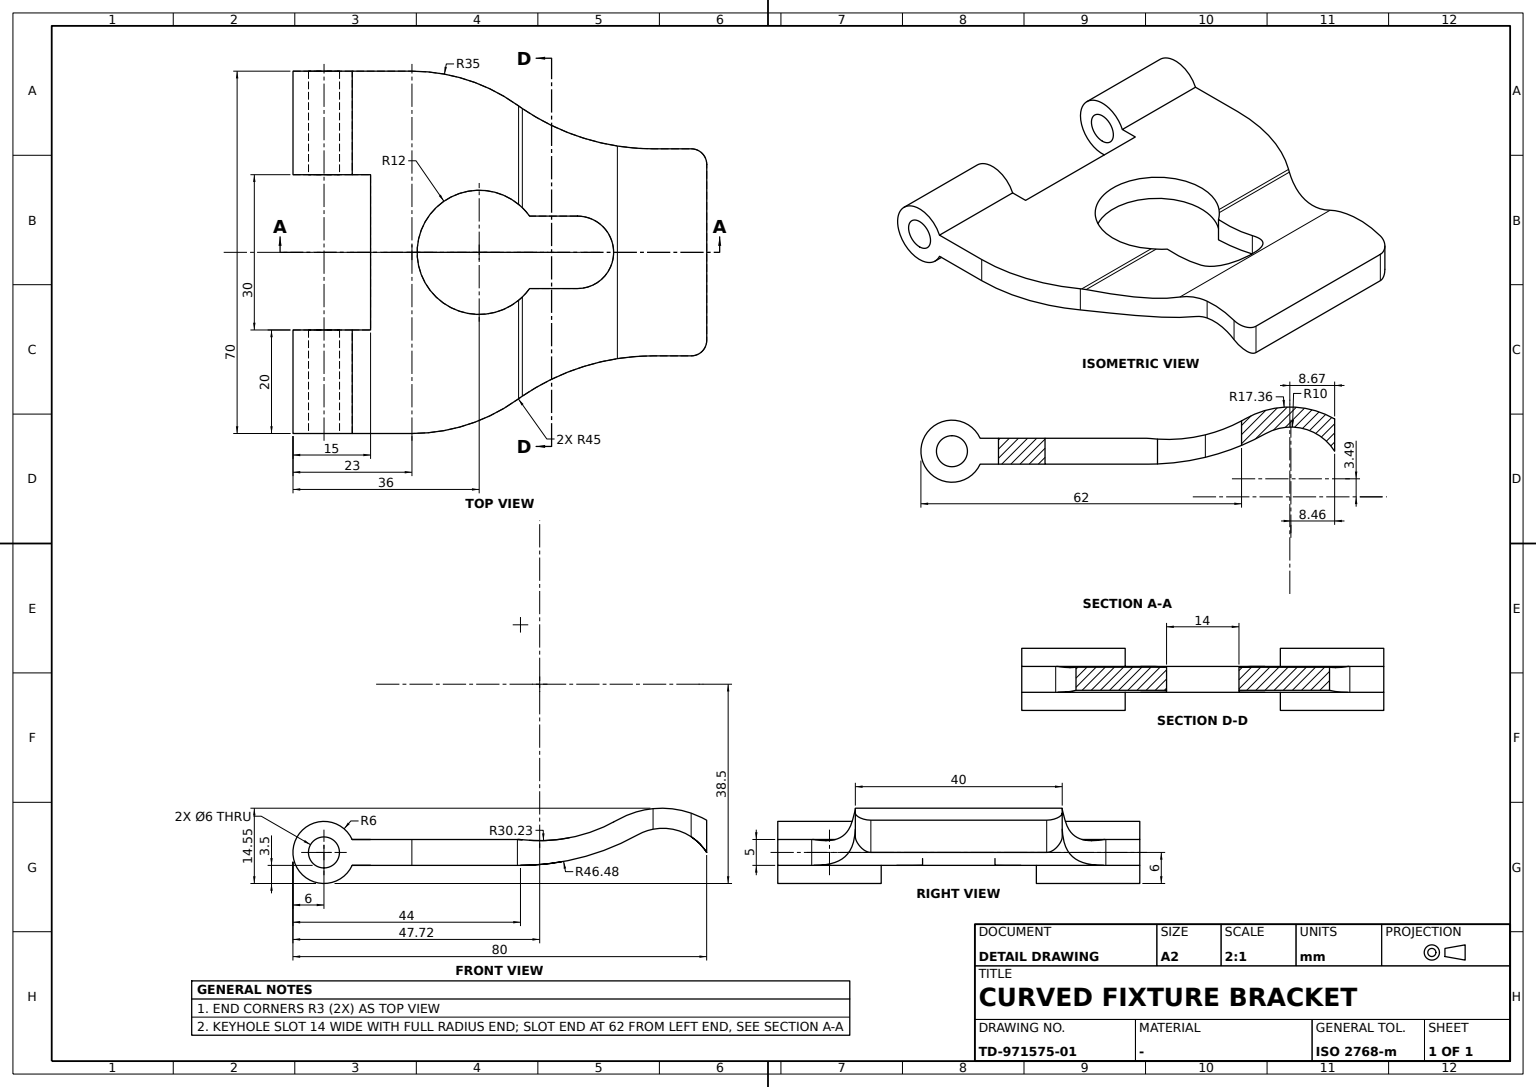
ISO-10303-21;
HEADER;
FILE_DESCRIPTION((''),'2;1');
FILE_NAME('','',(''),(''),'','','');
FILE_SCHEMA(('AUTOMOTIVE_DESIGN'));
ENDSEC;
DATA;
#1=APPLICATION_CONTEXT('');
#2=PRODUCT_CONTEXT('',#1,'mechanical');
#3=PRODUCT('','','',(#2));
#4=PRODUCT_DEFINITION_FORMATION('','',#3);
#5=PRODUCT_DEFINITION_CONTEXT('',#1,'design');
#6=PRODUCT_DEFINITION('','',#4,#5);
#7=PRODUCT_DEFINITION_SHAPE('','',#6);
#8=(LENGTH_UNIT()NAMED_UNIT(*)SI_UNIT(.MILLI.,.METRE.));
#9=(NAMED_UNIT(*)PLANE_ANGLE_UNIT()SI_UNIT($,.RADIAN.));
#10=(NAMED_UNIT(*)SI_UNIT($,.STERADIAN.)SOLID_ANGLE_UNIT());
#11=UNCERTAINTY_MEASURE_WITH_UNIT(LENGTH_MEASURE(0.005),#8,'distance_accuracy_value','');
#12=(GEOMETRIC_REPRESENTATION_CONTEXT(3)GLOBAL_UNCERTAINTY_ASSIGNED_CONTEXT((#11))GLOBAL_UNIT_ASSIGNED_CONTEXT((#8,#9,#10))REPRESENTATION_CONTEXT('',''));
#13=CARTESIAN_POINT('',(-28.4375,-36.596358,-2.5));
#14=VERTEX_POINT('',#13);
#15=CARTESIAN_POINT('',(-35.,-57.,-2.5));
#16=VERTEX_POINT('',#15);
#17=CARTESIAN_POINT('',(0.,-57.,-2.5));
#18=DIRECTION('',(0.,0.,1.));
#19=DIRECTION('',(1.,0.,0.));
#20=AXIS2_PLACEMENT_3D('',#17,#18,#19);
#21=CIRCLE('',#20,35.);
#22=EDGE_CURVE('',#14,#16,#21,.T.);
#23=ORIENTED_EDGE('',*,*,#22,.T.);
#24=CARTESIAN_POINT('',(-35.,-57.,2.5));
#25=VERTEX_POINT('',#24);
#26=CARTESIAN_POINT('',(-35.,-57.,0.));
#27=VECTOR('',#18,1000.);
#28=LINE('',#26,#27);
#29=EDGE_CURVE('',#16,#25,#28,.T.);
#30=ORIENTED_EDGE('',*,*,#29,.T.);
#31=CARTESIAN_POINT('',(-28.4375,-36.596358,2.5));
#32=VERTEX_POINT('',#31);
#33=CARTESIAN_POINT('',(0.,-57.,2.5));
#34=DIRECTION('',(0.,0.,-1.));
#35=DIRECTION('',(-1.,0.,0.));
#36=AXIS2_PLACEMENT_3D('',#33,#34,#35);
#37=CIRCLE('',#36,35.);
#38=EDGE_CURVE('',#25,#32,#37,.T.);
#39=ORIENTED_EDGE('',*,*,#38,.T.);
#40=CARTESIAN_POINT('',(-28.4375,-36.596358,0.));
#41=LINE('',#40,#27);
#42=EDGE_CURVE('',#14,#32,#41,.T.);
#43=ORIENTED_EDGE('',*,*,#42,.F.);
#44=EDGE_LOOP('',(#23,#30,#39,#43));
#45=FACE_BOUND('',#44,.T.);
#46=CARTESIAN_POINT('',(0.,-57.,0.));
#47=AXIS2_PLACEMENT_3D('',#46,#18,#19);
#48=CYLINDRICAL_SURFACE('',#47,35.);
#49=ADVANCED_FACE('',(#45),#48,.T.);
#50=CARTESIAN_POINT('',(-28.016901,-36.,-2.5));
#51=VERTEX_POINT('',#50);
#52=CARTESIAN_POINT('',(-65.,-10.363105,-2.5));
#53=AXIS2_PLACEMENT_3D('',#52,#18,#19);
#54=CIRCLE('',#53,45.);
#55=EDGE_CURVE('',#14,#51,#54,.T.);
#56=ORIENTED_EDGE('',*,*,#55,.F.);
#57=ORIENTED_EDGE('',*,*,#42,.T.);
#58=CARTESIAN_POINT('',(-28.283906,-36.380954,2.5));
#59=VERTEX_POINT('',#58);
#60=CARTESIAN_POINT('',(-65.,-10.363105,2.5));
#61=AXIS2_PLACEMENT_3D('',#60,#34,#35);
#62=CIRCLE('',#61,45.);
#63=EDGE_CURVE('',#59,#32,#62,.T.);
#64=ORIENTED_EDGE('',*,*,#63,.F.);
#65=CARTESIAN_POINT('',(-27.781293,-35.656737,2.459472));
#66=VERTEX_POINT('',#65);
#67=CARTESIAN_POINT('',(-27.946111,-35.899262,2.486701));
#68=CARTESIAN_POINT('',(-28.113645,-36.140683,2.5));
#69=B_SPLINE_CURVE_WITH_KNOTS('',3,(#65,#67,#68,#58),.UNSPECIFIED.,.F.,.F.,(4,4),(0.,0.00088247),.UNSPECIFIED.);
#70=EDGE_CURVE('',#66,#59,#69,.T.);
#71=ORIENTED_EDGE('',*,*,#70,.F.);
#72=CARTESIAN_POINT('',(-20.535037,-17.281708,6.256147));
#73=VERTEX_POINT('',#72);
#74=CARTESIAN_POINT('',(-20.766814,-18.771309,5.404617));
#75=CARTESIAN_POINT('',(-21.390954,-21.813993,3.995167));
#76=CARTESIAN_POINT('',(-23.441277,-28.200086,2.238521));
#77=CARTESIAN_POINT('',(-25.845824,-32.808762,2.139722));
#78=B_SPLINE_CURVE_WITH_KNOTS('',3,(#72,#74,#75,#76,#77,#65),.UNSPECIFIED.,.F.,.F.,(4,1,1,4),(0.,0.005116503,0.010233007,0.020466013),.UNSPECIFIED.);
#79=EDGE_CURVE('',#73,#66,#78,.T.);
#80=ORIENTED_EDGE('',*,*,#79,.F.);
#81=CARTESIAN_POINT('',(-20.,-10.363105,8.461947));
#82=VERTEX_POINT('',#81);
#83=CARTESIAN_POINT('',(-20.205135,-15.161472,7.46818));
#84=CARTESIAN_POINT('',(-20.,-12.817021,8.220804));
#85=B_SPLINE_CURVE_WITH_KNOTS('',3,(#72,#83,#84,#81),.UNSPECIFIED.,.F.,.F.,(4,4),(0.,0.007291634),.UNSPECIFIED.);
#86=EDGE_CURVE('',#73,#82,#85,.T.);
#87=ORIENTED_EDGE('',*,*,#86,.T.);
#88=CARTESIAN_POINT('',(-20.,-10.363105,4.486691));
#89=VERTEX_POINT('',#88);
#90=CARTESIAN_POINT('',(-20.,-10.363105,0.));
#91=LINE('',#90,#27);
#92=EDGE_CURVE('',#89,#82,#91,.T.);
#93=ORIENTED_EDGE('',*,*,#92,.F.);
#94=CARTESIAN_POINT('',(-20.098366,-13.336862,3.399904));
#95=VERTEX_POINT('',#94);
#96=CARTESIAN_POINT('',(-20.036616,-12.404486,3.920648));
#97=CARTESIAN_POINT('',(-20.,-11.413451,4.283158));
#98=B_SPLINE_CURVE_WITH_KNOTS('',3,(#94,#96,#97,#88),.UNSPECIFIED.,.F.,.F.,(4,4),(0.,0.003167651),.UNSPECIFIED.);
#99=EDGE_CURVE('',#95,#89,#98,.T.);
#100=ORIENTED_EDGE('',*,*,#99,.F.);
#101=CARTESIAN_POINT('',(-20.221084,-15.189824,2.365002));
#102=CARTESIAN_POINT('',(-20.6967,-18.956801,0.58839));
#103=CARTESIAN_POINT('',(-22.765086,-26.825025,-1.902632));
#104=CARTESIAN_POINT('',(-25.595054,-32.506308,-2.5));
#105=B_SPLINE_CURVE_WITH_KNOTS('',3,(#94,#101,#102,#103,#104,#50),.UNSPECIFIED.,.F.,.F.,(4,1,1,4),(0.,0.006286934,0.012573868,0.025147736),.UNSPECIFIED.);
#106=EDGE_CURVE('',#95,#51,#105,.T.);
#107=ORIENTED_EDGE('',*,*,#106,.T.);
#108=EDGE_LOOP('',(#56,#57,#64,#71,#80,#87,#93,#100,#107));
#109=FACE_BOUND('',#108,.T.);
#110=CARTESIAN_POINT('',(-65.,-10.363105,0.));
#111=AXIS2_PLACEMENT_3D('',#110,#18,#19);
#112=CYLINDRICAL_SURFACE('',#111,45.);
#113=ADVANCED_FACE('',(#109),#112,.F.);
#114=CARTESIAN_POINT('',(35.,-74.,-3.));
#115=VERTEX_POINT('',#114);
#116=CARTESIAN_POINT('',(35.,-74.,0.));
#117=AXIS2_PLACEMENT_3D('',#116,#19,#34);
#118=CIRCLE('',#117,3.);
#119=EDGE_CURVE('',#115,#115,#118,.T.);
#120=ORIENTED_EDGE('',*,*,#119,.F.);
#121=EDGE_LOOP('',(#120));
#122=FACE_BOUND('',#121,.T.);
#123=CARTESIAN_POINT('',(35.,-68.545644,2.5));
#124=VERTEX_POINT('',#123);
#125=CARTESIAN_POINT('',(35.,-57.,2.5));
#126=VERTEX_POINT('',#125);
#127=CARTESIAN_POINT('',(35.,-80.,2.5));
#128=DIRECTION('',(0.,1.,0.));
#129=VECTOR('',#128,1000.);
#130=LINE('',#127,#129);
#131=EDGE_CURVE('',#124,#126,#130,.T.);
#132=ORIENTED_EDGE('',*,*,#131,.F.);
#133=CARTESIAN_POINT('',(35.,-68.545644,-2.5));
#134=VERTEX_POINT('',#133);
#135=CIRCLE('',#117,6.);
#136=EDGE_CURVE('',#124,#134,#135,.T.);
#137=ORIENTED_EDGE('',*,*,#136,.T.);
#138=CARTESIAN_POINT('',(35.,-57.,-2.5));
#139=VERTEX_POINT('',#138);
#140=CARTESIAN_POINT('',(35.,-36.,-2.5));
#141=LINE('',#140,#129);
#142=EDGE_CURVE('',#134,#139,#141,.T.);
#143=ORIENTED_EDGE('',*,*,#142,.T.);
#144=CARTESIAN_POINT('',(35.,-57.,0.));
#145=LINE('',#144,#27);
#146=EDGE_CURVE('',#139,#126,#145,.T.);
#147=ORIENTED_EDGE('',*,*,#146,.T.);
#148=EDGE_LOOP('',(#132,#137,#143,#147));
#149=FACE_BOUND('',#148,.T.);
#150=CARTESIAN_POINT('',(35.,-80.,0.));
#151=AXIS2_PLACEMENT_3D('',#150,#19,#128);
#152=PLANE('',#151);
#153=ADVANCED_FACE('',(#122,#149),#152,.T.);
#154=CARTESIAN_POINT('',(7.,-34.253206,-2.467163));
#155=VERTEX_POINT('',#154);
#156=CARTESIAN_POINT('',(7.,-25.,-1.17954));
#157=VERTEX_POINT('',#156);
#158=CARTESIAN_POINT('',(7.,-36.,43.977594));
#159=AXIS2_PLACEMENT_3D('',#158,#19,#34);
#160=CIRCLE('',#159,46.477594);
#161=EDGE_CURVE('',#155,#157,#160,.T.);
#162=ORIENTED_EDGE('',*,*,#161,.F.);
#163=CARTESIAN_POINT('',(7.,-34.253206,2.334939));
#164=VERTEX_POINT('',#163);
#165=LINE('',#163,#27);
#166=EDGE_CURVE('',#164,#155,#165,.F.);
#167=ORIENTED_EDGE('',*,*,#166,.F.);
#168=CARTESIAN_POINT('',(7.,-25.,3.161425));
#169=VERTEX_POINT('',#168);
#170=CARTESIAN_POINT('',(7.,-32.284002,32.5));
#171=AXIS2_PLACEMENT_3D('',#170,#19,#34);
#172=CIRCLE('',#171,30.229268);
#173=EDGE_CURVE('',#164,#169,#172,.T.);
#174=ORIENTED_EDGE('',*,*,#173,.T.);
#175=CARTESIAN_POINT('',(7.,-25.,2.5));
#176=LINE('',#175,#27);
#177=EDGE_CURVE('',#169,#157,#176,.F.);
#178=ORIENTED_EDGE('',*,*,#177,.T.);
#179=EDGE_LOOP('',(#162,#167,#174,#178));
#180=FACE_BOUND('',#179,.T.);
#181=DIRECTION('',(0.,-1.,0.));
#182=AXIS2_PLACEMENT_3D('',#175,#19,#181);
#183=PLANE('',#182);
#184=ADVANCED_FACE('',(#180),#183,.F.);
#185=ORIENTED_EDGE('',*,*,#177,.F.);
#186=CARTESIAN_POINT('',(-7.,-25.,3.161425));
#187=VERTEX_POINT('',#186);
#188=CARTESIAN_POINT('',(7.,-23.145041,3.621963));
#189=CARTESIAN_POINT('',(5.894148,-20.513201,4.593679));
#190=CARTESIAN_POINT('',(2.843282,-18.399578,5.639759));
#191=CARTESIAN_POINT('',(0.017442,-17.803119,5.966173));
#192=CARTESIAN_POINT('',(-2.822505,-18.388043,5.645776));
#193=CARTESIAN_POINT('',(-5.895813,-20.509303,4.594871));
#194=CARTESIAN_POINT('',(-7.,-23.144084,3.622201));
#195=B_SPLINE_CURVE_WITH_KNOTS('',3,(#168,#188,#189,#190,#191,#192,#193,#194,#186),.UNSPECIFIED.,.F.,.F.,(4,1,1,1,1,1,4),(0.,0.005648977,0.008473466,0.011297955,0.014122443,0.016946932,0.022595909),.UNSPECIFIED.);
#196=EDGE_CURVE('',#169,#187,#195,.T.);
#197=ORIENTED_EDGE('',*,*,#196,.T.);
#198=CARTESIAN_POINT('',(-7.,-25.,-1.17954));
#199=VERTEX_POINT('',#198);
#200=CARTESIAN_POINT('',(-7.,-25.,2.5));
#201=LINE('',#200,#27);
#202=EDGE_CURVE('',#187,#199,#201,.F.);
#203=ORIENTED_EDGE('',*,*,#202,.T.);
#204=CARTESIAN_POINT('',(7.,-23.158455,-0.730951));
#205=CARTESIAN_POINT('',(5.557736,-19.611638,0.413862));
#206=CARTESIAN_POINT('',(0.017307,-17.196494,1.482838));
#207=CARTESIAN_POINT('',(-5.55843,-19.602443,0.41723));
#208=CARTESIAN_POINT('',(-7.,-23.158077,-0.730859));
#209=B_SPLINE_CURVE_WITH_KNOTS('',3,(#156,#204,#205,#206,#207,#208,#198),.UNSPECIFIED.,.F.,.F.,(4,1,1,1,4),(0.,0.005603851,0.011207701,0.016811552,0.022415402),.UNSPECIFIED.);
#210=EDGE_CURVE('',#157,#199,#209,.T.);
#211=ORIENTED_EDGE('',*,*,#210,.F.);
#212=EDGE_LOOP('',(#185,#197,#203,#211));
#213=FACE_BOUND('',#212,.T.);
#214=CARTESIAN_POINT('',(0.,-25.,2.5));
#215=AXIS2_PLACEMENT_3D('',#214,#18,#19);
#216=CYLINDRICAL_SURFACE('',#215,7.);
#217=ADVANCED_FACE('',(#213),#216,.F.);
#218=CARTESIAN_POINT('',(20.,-3.,3.046695));
#219=VERTEX_POINT('',#218);
#220=CARTESIAN_POINT('',(17.,0.,0.));
#221=VERTEX_POINT('',#220);
#222=CARTESIAN_POINT('',(20.,-2.198406,2.524184));
#223=CARTESIAN_POINT('',(19.550963,-1.160729,1.589565));
#224=CARTESIAN_POINT('',(18.372044,-0.239434,0.388292));
#225=CARTESIAN_POINT('',(17.4814,0.,0.));
#226=B_SPLINE_CURVE_WITH_KNOTS('',3,(#218,#222,#223,#224,#225,#220),.UNSPECIFIED.,.F.,.F.,(4,1,1,4),(0.,0.002824248,0.004236372,0.005648496),.UNSPECIFIED.);
#227=EDGE_CURVE('',#219,#221,#226,.T.);
#228=ORIENTED_EDGE('',*,*,#227,.T.);
#229=CARTESIAN_POINT('',(17.,0.,6.228303));
#230=VERTEX_POINT('',#229);
#231=CARTESIAN_POINT('',(17.,0.,4.272588));
#232=LINE('',#231,#27);
#233=EDGE_CURVE('',#221,#230,#232,.T.);
#234=ORIENTED_EDGE('',*,*,#233,.T.);
#235=CARTESIAN_POINT('',(20.,-3.,7.594938));
#236=VERTEX_POINT('',#235);
#237=CARTESIAN_POINT('',(17.830908,0.,6.228303));
#238=CARTESIAN_POINT('',(19.396375,-0.719594,6.66139));
#239=CARTESIAN_POINT('',(20.,-2.2162,7.324385));
#240=B_SPLINE_CURVE_WITH_KNOTS('',3,(#229,#237,#238,#239,#235),.UNSPECIFIED.,.F.,.F.,(4,1,4),(0.,0.002454286,0.004908571),.UNSPECIFIED.);
#241=EDGE_CURVE('',#230,#236,#240,.T.);
#242=ORIENTED_EDGE('',*,*,#241,.T.);
#243=CARTESIAN_POINT('',(20.,-3.,4.272588));
#244=LINE('',#243,#27);
#245=EDGE_CURVE('',#219,#236,#244,.T.);
#246=ORIENTED_EDGE('',*,*,#245,.F.);
#247=EDGE_LOOP('',(#228,#234,#242,#246));
#248=FACE_BOUND('',#247,.T.);
#249=CARTESIAN_POINT('',(17.,-3.,4.272588));
#250=AXIS2_PLACEMENT_3D('',#249,#18,#128);
#251=CYLINDRICAL_SURFACE('',#250,3.);
#252=ADVANCED_FACE('',(#248),#251,.T.);
#253=ORIENTED_EDGE('',*,*,#202,.F.);
#254=CARTESIAN_POINT('',(-7.,-34.253206,2.334939));
#255=VERTEX_POINT('',#254);
#256=CARTESIAN_POINT('',(-7.,-32.284002,32.5));
#257=AXIS2_PLACEMENT_3D('',#256,#35,#18);
#258=CIRCLE('',#257,30.229268);
#259=EDGE_CURVE('',#187,#255,#258,.T.);
#260=ORIENTED_EDGE('',*,*,#259,.T.);
#261=CARTESIAN_POINT('',(-7.,-34.253206,-2.467163));
#262=VERTEX_POINT('',#261);
#263=LINE('',#254,#27);
#264=EDGE_CURVE('',#255,#262,#263,.F.);
#265=ORIENTED_EDGE('',*,*,#264,.T.);
#266=CARTESIAN_POINT('',(-7.,-36.,43.977594));
#267=AXIS2_PLACEMENT_3D('',#266,#35,#18);
#268=CIRCLE('',#267,46.477594);
#269=EDGE_CURVE('',#199,#262,#268,.T.);
#270=ORIENTED_EDGE('',*,*,#269,.F.);
#271=EDGE_LOOP('',(#253,#260,#265,#270));
#272=FACE_BOUND('',#271,.T.);
#273=CARTESIAN_POINT('',(-7.,-34.253206,2.5));
#274=AXIS2_PLACEMENT_3D('',#273,#35,#128);
#275=PLANE('',#274);
#276=ADVANCED_FACE('',(#272),#275,.F.);
#277=CARTESIAN_POINT('',(-15.,-74.,3.));
#278=VERTEX_POINT('',#277);
#279=CARTESIAN_POINT('',(-15.,-74.,0.));
#280=AXIS2_PLACEMENT_3D('',#279,#35,#18);
#281=CIRCLE('',#280,3.);
#282=EDGE_CURVE('',#278,#278,#281,.T.);
#283=ORIENTED_EDGE('',*,*,#282,.T.);
#284=EDGE_LOOP('',(#283));
#285=FACE_BOUND('',#284,.T.);
#286=CARTESIAN_POINT('',(-15.,-68.545644,-2.5));
#287=VERTEX_POINT('',#286);
#288=CARTESIAN_POINT('',(-15.,-68.545644,2.5));
#289=VERTEX_POINT('',#288);
#290=CIRCLE('',#280,6.);
#291=EDGE_CURVE('',#287,#289,#290,.T.);
#292=ORIENTED_EDGE('',*,*,#291,.F.);
#293=CARTESIAN_POINT('',(-15.,-65.,-2.5));
#294=VERTEX_POINT('',#293);
#295=LINE('',#293,#129);
#296=EDGE_CURVE('',#287,#294,#295,.T.);
#297=ORIENTED_EDGE('',*,*,#296,.T.);
#298=CARTESIAN_POINT('',(-15.,-65.,2.5));
#299=VERTEX_POINT('',#298);
#300=CARTESIAN_POINT('',(-15.,-65.,0.));
#301=LINE('',#300,#27);
#302=EDGE_CURVE('',#294,#299,#301,.T.);
#303=ORIENTED_EDGE('',*,*,#302,.T.);
#304=LINE('',#288,#129);
#305=EDGE_CURVE('',#289,#299,#304,.T.);
#306=ORIENTED_EDGE('',*,*,#305,.F.);
#307=EDGE_LOOP('',(#292,#297,#303,#306));
#308=FACE_BOUND('',#307,.T.);
#309=AXIS2_PLACEMENT_3D('',#300,#35,#181);
#310=PLANE('',#309);
#311=ADVANCED_FACE('',(#285,#308),#310,.F.);
#312=CARTESIAN_POINT('',(-20.,-3.,7.594938));
#313=VERTEX_POINT('',#312);
#314=CARTESIAN_POINT('',(-20.,-8.665118,-8.817049));
#315=AXIS2_PLACEMENT_3D('',#314,#35,#18);
#316=CIRCLE('',#315,17.362225);
#317=EDGE_CURVE('',#82,#313,#316,.T.);
#318=ORIENTED_EDGE('',*,*,#317,.T.);
#319=CARTESIAN_POINT('',(-20.,-3.,3.046695));
#320=VERTEX_POINT('',#319);
#321=CARTESIAN_POINT('',(-20.,-3.,4.272588));
#322=LINE('',#321,#27);
#323=EDGE_CURVE('',#320,#313,#322,.T.);
#324=ORIENTED_EDGE('',*,*,#323,.F.);
#325=CARTESIAN_POINT('',(-20.,-8.460719,-5.330688));
#326=AXIS2_PLACEMENT_3D('',#325,#35,#18);
#327=CIRCLE('',#326,10.);
#328=EDGE_CURVE('',#89,#320,#327,.T.);
#329=ORIENTED_EDGE('',*,*,#328,.F.);
#330=ORIENTED_EDGE('',*,*,#92,.T.);
#331=EDGE_LOOP('',(#318,#324,#329,#330));
#332=FACE_BOUND('',#331,.T.);
#333=CARTESIAN_POINT('',(-20.,0.,0.));
#334=AXIS2_PLACEMENT_3D('',#333,#35,#181);
#335=PLANE('',#334);
#336=ADVANCED_FACE('',(#332),#335,.T.);
#337=CARTESIAN_POINT('',(8.944272,-36.,-2.5));
#338=VERTEX_POINT('',#337);
#339=CARTESIAN_POINT('',(7.711796,-34.764407,-2.486389));
#340=CARTESIAN_POINT('',(8.35988,-35.34663,-2.5));
#341=B_SPLINE_CURVE_WITH_KNOTS('',3,(#154,#339,#340,#337),.UNSPECIFIED.,.F.,.F.,(4,4),(0.,0.002613917),.UNSPECIFIED.);
#342=EDGE_CURVE('',#155,#338,#341,.T.);
#343=ORIENTED_EDGE('',*,*,#342,.T.);
#344=CARTESIAN_POINT('',(-8.944272,-36.,-2.5));
#345=VERTEX_POINT('',#344);
#346=CARTESIAN_POINT('',(0.,-44.,-2.5));
#347=AXIS2_PLACEMENT_3D('',#346,#18,#19);
#348=CIRCLE('',#347,12.);
#349=EDGE_CURVE('',#345,#338,#348,.T.);
#350=ORIENTED_EDGE('',*,*,#349,.F.);
#351=CARTESIAN_POINT('',(-7.711796,-34.764407,-2.486389));
#352=CARTESIAN_POINT('',(-8.35988,-35.34663,-2.5));
#353=B_SPLINE_CURVE_WITH_KNOTS('',3,(#261,#351,#352,#344),.UNSPECIFIED.,.F.,.F.,(4,4),(0.,0.002613917),.UNSPECIFIED.);
#354=EDGE_CURVE('',#345,#262,#353,.F.);
#355=ORIENTED_EDGE('',*,*,#354,.T.);
#356=ORIENTED_EDGE('',*,*,#264,.F.);
#357=CARTESIAN_POINT('',(-8.624962,-35.656737,2.459472));
#358=VERTEX_POINT('',#357);
#359=CARTESIAN_POINT('',(-8.125996,-35.140925,2.401561));
#360=CARTESIAN_POINT('',(-7.584346,-34.672874,2.362336));
#361=B_SPLINE_CURVE_WITH_KNOTS('',3,(#357,#359,#360,#254),.UNSPECIFIED.,.F.,.F.,(4,4),(0.,0.002150793),.UNSPECIFIED.);
#362=EDGE_CURVE('',#255,#358,#361,.F.);
#363=ORIENTED_EDGE('',*,*,#362,.T.);
#364=CARTESIAN_POINT('',(-9.27093,-36.380954,2.5));
#365=VERTEX_POINT('',#364);
#366=CARTESIAN_POINT('',(-8.849688,-35.889051,2.485555));
#367=CARTESIAN_POINT('',(-9.065018,-36.130398,2.5));
#368=B_SPLINE_CURVE_WITH_KNOTS('',3,(#357,#366,#367,#364),.UNSPECIFIED.,.F.,.F.,(4,4),(0.,0.000971292),.UNSPECIFIED.);
#369=EDGE_CURVE('',#358,#365,#368,.T.);
#370=ORIENTED_EDGE('',*,*,#369,.T.);
#371=CARTESIAN_POINT('',(9.27093,-36.380954,2.5));
#372=VERTEX_POINT('',#371);
#373=CARTESIAN_POINT('',(0.,-44.,2.5));
#374=AXIS2_PLACEMENT_3D('',#373,#34,#35);
#375=CIRCLE('',#374,12.);
#376=EDGE_CURVE('',#372,#365,#375,.T.);
#377=ORIENTED_EDGE('',*,*,#376,.F.);
#378=CARTESIAN_POINT('',(8.624962,-35.656737,2.459472));
#379=VERTEX_POINT('',#378);
#380=CARTESIAN_POINT('',(8.849688,-35.889051,2.485555));
#381=CARTESIAN_POINT('',(9.065018,-36.130398,2.5));
#382=B_SPLINE_CURVE_WITH_KNOTS('',3,(#378,#380,#381,#371),.UNSPECIFIED.,.F.,.F.,(4,4),(0.,0.000971292),.UNSPECIFIED.);
#383=EDGE_CURVE('',#372,#379,#382,.F.);
#384=ORIENTED_EDGE('',*,*,#383,.T.);
#385=CARTESIAN_POINT('',(8.125996,-35.140925,2.401561));
#386=CARTESIAN_POINT('',(7.584346,-34.672874,2.362336));
#387=B_SPLINE_CURVE_WITH_KNOTS('',3,(#378,#385,#386,#163),.UNSPECIFIED.,.F.,.F.,(4,4),(0.,0.002150793),.UNSPECIFIED.);
#388=EDGE_CURVE('',#379,#164,#387,.T.);
#389=ORIENTED_EDGE('',*,*,#388,.T.);
#390=ORIENTED_EDGE('',*,*,#166,.T.);
#391=EDGE_LOOP('',(#343,#350,#355,#356,#363,#370,#377,#384,#389,#390));
#392=FACE_BOUND('',#391,.T.);
#393=AXIS2_PLACEMENT_3D('',#373,#18,#19);
#394=CYLINDRICAL_SURFACE('',#393,12.);
#395=ADVANCED_FACE('',(#392),#394,.F.);
#396=CARTESIAN_POINT('',(20.098366,-13.336862,3.399904));
#397=VERTEX_POINT('',#396);
#398=CARTESIAN_POINT('',(28.016901,-36.,-2.5));
#399=VERTEX_POINT('',#398);
#400=CARTESIAN_POINT('',(20.221084,-15.189824,2.365002));
#401=CARTESIAN_POINT('',(20.6967,-18.956801,0.58839));
#402=CARTESIAN_POINT('',(22.765086,-26.825025,-1.902632));
#403=CARTESIAN_POINT('',(25.595054,-32.506308,-2.5));
#404=B_SPLINE_CURVE_WITH_KNOTS('',3,(#396,#400,#401,#402,#403,#398),.UNSPECIFIED.,.F.,.F.,(4,1,1,4),(0.,0.006286934,0.012573868,0.025147736),.UNSPECIFIED.);
#405=EDGE_CURVE('',#397,#399,#404,.T.);
#406=ORIENTED_EDGE('',*,*,#405,.T.);
#407=CARTESIAN_POINT('',(0.,-36.,-2.5));
#408=VECTOR('',#19,1000.);
#409=LINE('',#407,#408);
#410=EDGE_CURVE('',#338,#399,#409,.T.);
#411=ORIENTED_EDGE('',*,*,#410,.F.);
#412=ORIENTED_EDGE('',*,*,#342,.F.);
#413=ORIENTED_EDGE('',*,*,#161,.T.);
#414=ORIENTED_EDGE('',*,*,#210,.T.);
#415=ORIENTED_EDGE('',*,*,#269,.T.);
#416=ORIENTED_EDGE('',*,*,#354,.F.);
#417=EDGE_CURVE('',#51,#345,#409,.T.);
#418=ORIENTED_EDGE('',*,*,#417,.F.);
#419=ORIENTED_EDGE('',*,*,#106,.F.);
#420=CARTESIAN_POINT('',(0.,-13.336862,3.399904));
#421=LINE('',#420,#408);
#422=EDGE_CURVE('',#95,#397,#421,.T.);
#423=ORIENTED_EDGE('',*,*,#422,.T.);
#424=EDGE_LOOP('',(#406,#411,#412,#413,#414,#415,#416,#418,#419,#423));
#425=FACE_BOUND('',#424,.T.);
#426=CARTESIAN_POINT('',(0.,-36.,43.977594));
#427=AXIS2_PLACEMENT_3D('',#426,#19,#128);
#428=CYLINDRICAL_SURFACE('',#427,46.477594);
#429=ADVANCED_FACE('',(#425),#428,.T.);
#430=CARTESIAN_POINT('',(-35.,-74.,-3.));
#431=VERTEX_POINT('',#430);
#432=CARTESIAN_POINT('',(-35.,-74.,0.));
#433=AXIS2_PLACEMENT_3D('',#432,#19,#34);
#434=CIRCLE('',#433,3.);
#435=EDGE_CURVE('',#431,#431,#434,.T.);
#436=ORIENTED_EDGE('',*,*,#435,.T.);
#437=EDGE_LOOP('',(#436));
#438=FACE_BOUND('',#437,.T.);
#439=ORIENTED_EDGE('',*,*,#29,.F.);
#440=CARTESIAN_POINT('',(-35.,-68.545644,-2.5));
#441=VERTEX_POINT('',#440);
#442=CARTESIAN_POINT('',(-35.,-36.,-2.5));
#443=LINE('',#442,#129);
#444=EDGE_CURVE('',#441,#16,#443,.T.);
#445=ORIENTED_EDGE('',*,*,#444,.F.);
#446=CARTESIAN_POINT('',(-35.,-68.545644,2.5));
#447=VERTEX_POINT('',#446);
#448=CIRCLE('',#433,6.);
#449=EDGE_CURVE('',#447,#441,#448,.T.);
#450=ORIENTED_EDGE('',*,*,#449,.F.);
#451=CARTESIAN_POINT('',(-35.,-80.,2.5));
#452=LINE('',#451,#129);
#453=EDGE_CURVE('',#447,#25,#452,.T.);
#454=ORIENTED_EDGE('',*,*,#453,.T.);
#455=EDGE_LOOP('',(#439,#445,#450,#454));
#456=FACE_BOUND('',#455,.T.);
#457=CARTESIAN_POINT('',(-35.,-80.,0.));
#458=AXIS2_PLACEMENT_3D('',#457,#19,#128);
#459=PLANE('',#458);
#460=ADVANCED_FACE('',(#438,#456),#459,.F.);
#461=ORIENTED_EDGE('',*,*,#388,.F.);
#462=CARTESIAN_POINT('',(27.781293,-35.656737,2.459472));
#463=VERTEX_POINT('',#462);
#464=CARTESIAN_POINT('',(18.203127,-35.656737,2.459472));
#465=LINE('',#464,#408);
#466=EDGE_CURVE('',#379,#463,#465,.T.);
#467=ORIENTED_EDGE('',*,*,#466,.T.);
#468=CARTESIAN_POINT('',(20.535037,-17.281708,6.256147));
#469=VERTEX_POINT('',#468);
#470=CARTESIAN_POINT('',(20.766814,-18.771309,5.404617));
#471=CARTESIAN_POINT('',(21.390954,-21.813993,3.995167));
#472=CARTESIAN_POINT('',(23.441277,-28.200086,2.238521));
#473=CARTESIAN_POINT('',(25.845824,-32.808762,2.139722));
#474=B_SPLINE_CURVE_WITH_KNOTS('',3,(#468,#470,#471,#472,#473,#462),.UNSPECIFIED.,.F.,.F.,(4,1,1,4),(0.,0.005116503,0.010233007,0.020466013),.UNSPECIFIED.);
#475=EDGE_CURVE('',#469,#463,#474,.T.);
#476=ORIENTED_EDGE('',*,*,#475,.F.);
#477=CARTESIAN_POINT('',(0.,-17.281708,6.256147));
#478=LINE('',#477,#408);
#479=EDGE_CURVE('',#73,#469,#478,.T.);
#480=ORIENTED_EDGE('',*,*,#479,.F.);
#481=ORIENTED_EDGE('',*,*,#79,.T.);
#482=CARTESIAN_POINT('',(-18.203127,-35.656737,2.459472));
#483=LINE('',#482,#408);
#484=EDGE_CURVE('',#66,#358,#483,.T.);
#485=ORIENTED_EDGE('',*,*,#484,.T.);
#486=ORIENTED_EDGE('',*,*,#362,.F.);
#487=ORIENTED_EDGE('',*,*,#259,.F.);
#488=ORIENTED_EDGE('',*,*,#196,.F.);
#489=ORIENTED_EDGE('',*,*,#173,.F.);
#490=EDGE_LOOP('',(#461,#467,#476,#480,#481,#485,#486,#487,#488,#489));
#491=FACE_BOUND('',#490,.T.);
#492=CARTESIAN_POINT('',(0.,-32.284002,32.5));
#493=AXIS2_PLACEMENT_3D('',#492,#19,#128);
#494=CYLINDRICAL_SURFACE('',#493,30.229268);
#495=ADVANCED_FACE('',(#491),#494,.F.);
#496=ORIENTED_EDGE('',*,*,#444,.T.);
#497=ORIENTED_EDGE('',*,*,#22,.F.);
#498=ORIENTED_EDGE('',*,*,#55,.T.);
#499=ORIENTED_EDGE('',*,*,#417,.T.);
#500=ORIENTED_EDGE('',*,*,#349,.T.);
#501=ORIENTED_EDGE('',*,*,#410,.T.);
#502=CARTESIAN_POINT('',(28.4375,-36.596358,-2.5));
#503=VERTEX_POINT('',#502);
#504=CARTESIAN_POINT('',(65.,-10.363105,-2.5));
#505=AXIS2_PLACEMENT_3D('',#504,#18,#19);
#506=CIRCLE('',#505,45.);
#507=EDGE_CURVE('',#399,#503,#506,.T.);
#508=ORIENTED_EDGE('',*,*,#507,.T.);
#509=EDGE_CURVE('',#139,#503,#21,.T.);
#510=ORIENTED_EDGE('',*,*,#509,.F.);
#511=ORIENTED_EDGE('',*,*,#142,.F.);
#512=CARTESIAN_POINT('',(15.,-68.545644,-2.5));
#513=VERTEX_POINT('',#512);
#514=LINE('',#512,#408);
#515=EDGE_CURVE('',#513,#134,#514,.T.);
#516=ORIENTED_EDGE('',*,*,#515,.F.);
#517=CARTESIAN_POINT('',(15.,-65.,-2.5));
#518=VERTEX_POINT('',#517);
#519=CARTESIAN_POINT('',(15.,-36.,-2.5));
#520=LINE('',#519,#129);
#521=EDGE_CURVE('',#513,#518,#520,.T.);
#522=ORIENTED_EDGE('',*,*,#521,.T.);
#523=CARTESIAN_POINT('',(0.,-65.,-2.5));
#524=VECTOR('',#35,1000.);
#525=LINE('',#523,#524);
#526=EDGE_CURVE('',#518,#294,#525,.T.);
#527=ORIENTED_EDGE('',*,*,#526,.T.);
#528=ORIENTED_EDGE('',*,*,#296,.F.);
#529=LINE('',#440,#408);
#530=EDGE_CURVE('',#441,#287,#529,.T.);
#531=ORIENTED_EDGE('',*,*,#530,.F.);
#532=EDGE_LOOP('',(#496,#497,#498,#499,#500,#501,#508,#510,#511,#516,#522,#527,#528,#531));
#533=FACE_BOUND('',#532,.T.);
#534=AXIS2_PLACEMENT_3D('',#407,#18,#181);
#535=PLANE('',#534);
#536=ADVANCED_FACE('',(#533),#535,.F.);
#537=CARTESIAN_POINT('',(15.,-74.,-3.));
#538=VERTEX_POINT('',#537);
#539=CARTESIAN_POINT('',(15.,-74.,0.));
#540=AXIS2_PLACEMENT_3D('',#539,#19,#34);
#541=CIRCLE('',#540,3.);
#542=EDGE_CURVE('',#538,#538,#541,.T.);
#543=ORIENTED_EDGE('',*,*,#542,.T.);
#544=EDGE_LOOP('',(#543));
#545=FACE_BOUND('',#544,.T.);
#546=ORIENTED_EDGE('',*,*,#521,.F.);
#547=CARTESIAN_POINT('',(15.,-68.545644,2.5));
#548=VERTEX_POINT('',#547);
#549=CIRCLE('',#540,6.);
#550=EDGE_CURVE('',#548,#513,#549,.T.);
#551=ORIENTED_EDGE('',*,*,#550,.F.);
#552=CARTESIAN_POINT('',(15.,-65.,2.5));
#553=VERTEX_POINT('',#552);
#554=CARTESIAN_POINT('',(15.,-80.,2.5));
#555=LINE('',#554,#129);
#556=EDGE_CURVE('',#548,#553,#555,.T.);
#557=ORIENTED_EDGE('',*,*,#556,.T.);
#558=CARTESIAN_POINT('',(15.,-65.,0.));
#559=LINE('',#558,#27);
#560=EDGE_CURVE('',#518,#553,#559,.T.);
#561=ORIENTED_EDGE('',*,*,#560,.F.);
#562=EDGE_LOOP('',(#546,#551,#557,#561));
#563=FACE_BOUND('',#562,.T.);
#564=CARTESIAN_POINT('',(15.,-80.,0.));
#565=AXIS2_PLACEMENT_3D('',#564,#19,#128);
#566=PLANE('',#565);
#567=ADVANCED_FACE('',(#545,#563),#566,.F.);
#568=ORIENTED_EDGE('',*,*,#86,.F.);
#569=ORIENTED_EDGE('',*,*,#479,.T.);
#570=CARTESIAN_POINT('',(20.,-10.363105,8.461947));
#571=VERTEX_POINT('',#570);
#572=CARTESIAN_POINT('',(20.205135,-15.161472,7.46818));
#573=CARTESIAN_POINT('',(20.,-12.817021,8.220804));
#574=B_SPLINE_CURVE_WITH_KNOTS('',3,(#468,#572,#573,#570),.UNSPECIFIED.,.F.,.F.,(4,4),(0.,0.007291634),.UNSPECIFIED.);
#575=EDGE_CURVE('',#469,#571,#574,.T.);
#576=ORIENTED_EDGE('',*,*,#575,.T.);
#577=CARTESIAN_POINT('',(20.,-8.665118,-8.817049));
#578=AXIS2_PLACEMENT_3D('',#577,#35,#18);
#579=CIRCLE('',#578,17.362225);
#580=EDGE_CURVE('',#571,#236,#579,.T.);
#581=ORIENTED_EDGE('',*,*,#580,.T.);
#582=ORIENTED_EDGE('',*,*,#241,.F.);
#583=CARTESIAN_POINT('',(-17.,0.,6.228303));
#584=VERTEX_POINT('',#583);
#585=LINE('',#583,#408);
#586=EDGE_CURVE('',#584,#230,#585,.T.);
#587=ORIENTED_EDGE('',*,*,#586,.F.);
#588=CARTESIAN_POINT('',(-17.830908,0.,6.228303));
#589=CARTESIAN_POINT('',(-19.396375,-0.719594,6.66139));
#590=CARTESIAN_POINT('',(-20.,-2.2162,7.324385));
#591=B_SPLINE_CURVE_WITH_KNOTS('',3,(#583,#588,#589,#590,#312),.UNSPECIFIED.,.F.,.F.,(4,1,4),(0.,0.002454286,0.004908571),.UNSPECIFIED.);
#592=EDGE_CURVE('',#584,#313,#591,.T.);
#593=ORIENTED_EDGE('',*,*,#592,.T.);
#594=ORIENTED_EDGE('',*,*,#317,.F.);
#595=EDGE_LOOP('',(#568,#569,#576,#581,#582,#587,#593,#594));
#596=FACE_BOUND('',#595,.T.);
#597=CARTESIAN_POINT('',(0.,-8.665118,-8.817049));
#598=AXIS2_PLACEMENT_3D('',#597,#19,#128);
#599=CYLINDRICAL_SURFACE('',#598,17.362225);
#600=ADVANCED_FACE('',(#596),#599,.T.);
#601=ORIENTED_EDGE('',*,*,#136,.F.);
#602=LINE('',#547,#408);
#603=EDGE_CURVE('',#548,#124,#602,.T.);
#604=ORIENTED_EDGE('',*,*,#603,.F.);
#605=ORIENTED_EDGE('',*,*,#550,.T.);
#606=ORIENTED_EDGE('',*,*,#515,.T.);
#607=EDGE_LOOP('',(#601,#604,#605,#606));
#608=FACE_BOUND('',#607,.T.);
#609=CARTESIAN_POINT('',(0.,-74.,0.));
#610=AXIS2_PLACEMENT_3D('',#609,#19,#128);
#611=CYLINDRICAL_SURFACE('',#610,6.);
#612=ADVANCED_FACE('',(#608),#611,.T.);
#613=LINE('',#446,#408);
#614=EDGE_CURVE('',#447,#289,#613,.T.);
#615=ORIENTED_EDGE('',*,*,#614,.F.);
#616=ORIENTED_EDGE('',*,*,#449,.T.);
#617=ORIENTED_EDGE('',*,*,#530,.T.);
#618=ORIENTED_EDGE('',*,*,#291,.T.);
#619=EDGE_LOOP('',(#615,#616,#617,#618));
#620=FACE_BOUND('',#619,.T.);
#621=ADVANCED_FACE('',(#620),#611,.T.);
#622=CARTESIAN_POINT('',(28.283906,-36.380954,2.5));
#623=VERTEX_POINT('',#622);
#624=CARTESIAN_POINT('',(27.946111,-35.899262,2.486701));
#625=CARTESIAN_POINT('',(28.113645,-36.140683,2.5));
#626=B_SPLINE_CURVE_WITH_KNOTS('',3,(#462,#624,#625,#622),.UNSPECIFIED.,.F.,.F.,(4,4),(0.,0.00088247),.UNSPECIFIED.);
#627=EDGE_CURVE('',#463,#623,#626,.T.);
#628=ORIENTED_EDGE('',*,*,#627,.F.);
#629=ORIENTED_EDGE('',*,*,#466,.F.);
#630=ORIENTED_EDGE('',*,*,#383,.F.);
#631=CARTESIAN_POINT('',(0.,-36.380954,2.5));
#632=LINE('',#631,#408);
#633=EDGE_CURVE('',#372,#623,#632,.T.);
#634=ORIENTED_EDGE('',*,*,#633,.T.);
#635=EDGE_LOOP('',(#628,#629,#630,#634));
#636=FACE_BOUND('',#635,.T.);
#637=CARTESIAN_POINT('',(0.,-36.380954,-3.991037));
#638=AXIS2_PLACEMENT_3D('',#637,#19,#128);
#639=CYLINDRICAL_SURFACE('',#638,6.491037);
#640=ADVANCED_FACE('',(#636),#639,.T.);
#641=ORIENTED_EDGE('',*,*,#580,.F.);
#642=CARTESIAN_POINT('',(20.,-10.363105,4.486691));
#643=VERTEX_POINT('',#642);
#644=CARTESIAN_POINT('',(20.,-10.363105,0.));
#645=LINE('',#644,#27);
#646=EDGE_CURVE('',#643,#571,#645,.T.);
#647=ORIENTED_EDGE('',*,*,#646,.F.);
#648=CARTESIAN_POINT('',(20.,-8.460719,-5.330688));
#649=AXIS2_PLACEMENT_3D('',#648,#35,#18);
#650=CIRCLE('',#649,10.);
#651=EDGE_CURVE('',#643,#219,#650,.T.);
#652=ORIENTED_EDGE('',*,*,#651,.T.);
#653=ORIENTED_EDGE('',*,*,#245,.T.);
#654=EDGE_LOOP('',(#641,#647,#652,#653));
#655=FACE_BOUND('',#654,.T.);
#656=CARTESIAN_POINT('',(20.,0.,0.));
#657=AXIS2_PLACEMENT_3D('',#656,#35,#181);
#658=PLANE('',#657);
#659=ADVANCED_FACE('',(#655),#658,.F.);
#660=CARTESIAN_POINT('',(-17.,0.,0.));
#661=VERTEX_POINT('',#660);
#662=CARTESIAN_POINT('',(-17.,0.,4.272588));
#663=LINE('',#662,#27);
#664=EDGE_CURVE('',#661,#584,#663,.T.);
#665=ORIENTED_EDGE('',*,*,#664,.F.);
#666=CARTESIAN_POINT('',(-20.,-2.198406,2.524184));
#667=CARTESIAN_POINT('',(-19.550963,-1.160729,1.589565));
#668=CARTESIAN_POINT('',(-18.372044,-0.239434,0.388292));
#669=CARTESIAN_POINT('',(-17.4814,0.,0.));
#670=B_SPLINE_CURVE_WITH_KNOTS('',3,(#319,#666,#667,#668,#669,#660),.UNSPECIFIED.,.F.,.F.,(4,1,1,4),(0.,0.002824248,0.004236372,0.005648496),.UNSPECIFIED.);
#671=EDGE_CURVE('',#320,#661,#670,.T.);
#672=ORIENTED_EDGE('',*,*,#671,.F.);
#673=ORIENTED_EDGE('',*,*,#323,.T.);
#674=ORIENTED_EDGE('',*,*,#592,.F.);
#675=EDGE_LOOP('',(#665,#672,#673,#674));
#676=FACE_BOUND('',#675,.T.);
#677=CARTESIAN_POINT('',(-17.,-3.,4.272588));
#678=AXIS2_PLACEMENT_3D('',#677,#18,#35);
#679=CYLINDRICAL_SURFACE('',#678,3.);
#680=ADVANCED_FACE('',(#676),#679,.T.);
#681=LINE('',#660,#408);
#682=EDGE_CURVE('',#661,#221,#681,.T.);
#683=ORIENTED_EDGE('',*,*,#682,.F.);
#684=ORIENTED_EDGE('',*,*,#664,.T.);
#685=ORIENTED_EDGE('',*,*,#586,.T.);
#686=ORIENTED_EDGE('',*,*,#233,.F.);
#687=EDGE_LOOP('',(#683,#684,#685,#686));
#688=FACE_BOUND('',#687,.T.);
#689=AXIS2_PLACEMENT_3D('',#333,#181,#19);
#690=PLANE('',#689);
#691=ADVANCED_FACE('',(#688),#690,.F.);
#692=ORIENTED_EDGE('',*,*,#542,.F.);
#693=EDGE_LOOP('',(#692));
#694=FACE_BOUND('',#693,.T.);
#695=ORIENTED_EDGE('',*,*,#119,.T.);
#696=EDGE_LOOP('',(#695));
#697=FACE_BOUND('',#696,.T.);
#698=CYLINDRICAL_SURFACE('',#610,3.);
#699=ADVANCED_FACE('',(#694,#697),#698,.F.);
#700=CARTESIAN_POINT('',(20.036616,-12.404486,3.920648));
#701=CARTESIAN_POINT('',(20.,-11.413451,4.283158));
#702=B_SPLINE_CURVE_WITH_KNOTS('',3,(#396,#700,#701,#642),.UNSPECIFIED.,.F.,.F.,(4,4),(0.,0.003167651),.UNSPECIFIED.);
#703=EDGE_CURVE('',#397,#643,#702,.T.);
#704=ORIENTED_EDGE('',*,*,#703,.F.);
#705=ORIENTED_EDGE('',*,*,#422,.F.);
#706=ORIENTED_EDGE('',*,*,#99,.T.);
#707=ORIENTED_EDGE('',*,*,#328,.T.);
#708=ORIENTED_EDGE('',*,*,#671,.T.);
#709=ORIENTED_EDGE('',*,*,#682,.T.);
#710=ORIENTED_EDGE('',*,*,#227,.F.);
#711=ORIENTED_EDGE('',*,*,#651,.F.);
#712=EDGE_LOOP('',(#704,#705,#706,#707,#708,#709,#710,#711));
#713=FACE_BOUND('',#712,.T.);
#714=CARTESIAN_POINT('',(0.,-8.460719,-5.330688));
#715=AXIS2_PLACEMENT_3D('',#714,#19,#128);
#716=CYLINDRICAL_SURFACE('',#715,10.);
#717=ADVANCED_FACE('',(#713),#716,.F.);
#718=ORIENTED_EDGE('',*,*,#509,.T.);
#719=CARTESIAN_POINT('',(28.4375,-36.596358,2.5));
#720=VERTEX_POINT('',#719);
#721=CARTESIAN_POINT('',(28.4375,-36.596358,0.));
#722=LINE('',#721,#27);
#723=EDGE_CURVE('',#503,#720,#722,.T.);
#724=ORIENTED_EDGE('',*,*,#723,.T.);
#725=EDGE_CURVE('',#720,#126,#37,.T.);
#726=ORIENTED_EDGE('',*,*,#725,.T.);
#727=ORIENTED_EDGE('',*,*,#146,.F.);
#728=EDGE_LOOP('',(#718,#724,#726,#727));
#729=FACE_BOUND('',#728,.T.);
#730=ADVANCED_FACE('',(#729),#48,.T.);
#731=ORIENTED_EDGE('',*,*,#369,.F.);
#732=ORIENTED_EDGE('',*,*,#484,.F.);
#733=ORIENTED_EDGE('',*,*,#70,.T.);
#734=EDGE_CURVE('',#59,#365,#632,.T.);
#735=ORIENTED_EDGE('',*,*,#734,.T.);
#736=EDGE_LOOP('',(#731,#732,#733,#735));
#737=FACE_BOUND('',#736,.T.);
#738=ADVANCED_FACE('',(#737),#639,.T.);
#739=ORIENTED_EDGE('',*,*,#282,.F.);
#740=EDGE_LOOP('',(#739));
#741=FACE_BOUND('',#740,.T.);
#742=ORIENTED_EDGE('',*,*,#435,.F.);
#743=EDGE_LOOP('',(#742));
#744=FACE_BOUND('',#743,.T.);
#745=ADVANCED_FACE('',(#741,#744),#698,.F.);
#746=ORIENTED_EDGE('',*,*,#526,.F.);
#747=ORIENTED_EDGE('',*,*,#560,.T.);
#748=LINE('',#552,#524);
#749=EDGE_CURVE('',#553,#299,#748,.T.);
#750=ORIENTED_EDGE('',*,*,#749,.T.);
#751=ORIENTED_EDGE('',*,*,#302,.F.);
#752=EDGE_LOOP('',(#746,#747,#750,#751));
#753=FACE_BOUND('',#752,.T.);
#754=AXIS2_PLACEMENT_3D('',#558,#128,#35);
#755=PLANE('',#754);
#756=ADVANCED_FACE('',(#753),#755,.F.);
#757=CARTESIAN_POINT('',(65.,-10.363105,2.5));
#758=AXIS2_PLACEMENT_3D('',#757,#34,#35);
#759=CIRCLE('',#758,45.);
#760=EDGE_CURVE('',#720,#623,#759,.T.);
#761=ORIENTED_EDGE('',*,*,#760,.F.);
#762=ORIENTED_EDGE('',*,*,#723,.F.);
#763=ORIENTED_EDGE('',*,*,#507,.F.);
#764=ORIENTED_EDGE('',*,*,#405,.F.);
#765=ORIENTED_EDGE('',*,*,#703,.T.);
#766=ORIENTED_EDGE('',*,*,#646,.T.);
#767=ORIENTED_EDGE('',*,*,#575,.F.);
#768=ORIENTED_EDGE('',*,*,#475,.T.);
#769=ORIENTED_EDGE('',*,*,#627,.T.);
#770=EDGE_LOOP('',(#761,#762,#763,#764,#765,#766,#767,#768,#769));
#771=FACE_BOUND('',#770,.T.);
#772=CARTESIAN_POINT('',(65.,-10.363105,0.));
#773=AXIS2_PLACEMENT_3D('',#772,#18,#19);
#774=CYLINDRICAL_SURFACE('',#773,45.);
#775=ADVANCED_FACE('',(#771),#774,.F.);
#776=ORIENTED_EDGE('',*,*,#603,.T.);
#777=ORIENTED_EDGE('',*,*,#131,.T.);
#778=ORIENTED_EDGE('',*,*,#725,.F.);
#779=ORIENTED_EDGE('',*,*,#760,.T.);
#780=ORIENTED_EDGE('',*,*,#633,.F.);
#781=ORIENTED_EDGE('',*,*,#376,.T.);
#782=ORIENTED_EDGE('',*,*,#734,.F.);
#783=ORIENTED_EDGE('',*,*,#63,.T.);
#784=ORIENTED_EDGE('',*,*,#38,.F.);
#785=ORIENTED_EDGE('',*,*,#453,.F.);
#786=ORIENTED_EDGE('',*,*,#614,.T.);
#787=ORIENTED_EDGE('',*,*,#305,.T.);
#788=ORIENTED_EDGE('',*,*,#749,.F.);
#789=ORIENTED_EDGE('',*,*,#556,.F.);
#790=EDGE_LOOP('',(#776,#777,#778,#779,#780,#781,#782,#783,#784,#785,#786,#787,#788,#789));
#791=FACE_BOUND('',#790,.T.);
#792=CARTESIAN_POINT('',(0.,-68.545644,2.5));
#793=AXIS2_PLACEMENT_3D('',#792,#34,#128);
#794=PLANE('',#793);
#795=ADVANCED_FACE('',(#791),#794,.F.);
#796=CLOSED_SHELL('',(#49,#113,#153,#184,#217,#252,#276,#311,#336,#395,#429,#460,#495,#536,#567,#600,#612,#621,#640,#659,#680,#691,#699,#717,#730,#738,#745,#756,#775,#795));
#797=MANIFOLD_SOLID_BREP('',#796);
#798=ADVANCED_BREP_SHAPE_REPRESENTATION('',(#797),#12);
#799=SHAPE_DEFINITION_REPRESENTATION(#7,#798);
ENDSEC;
END-ISO-10303-21;
